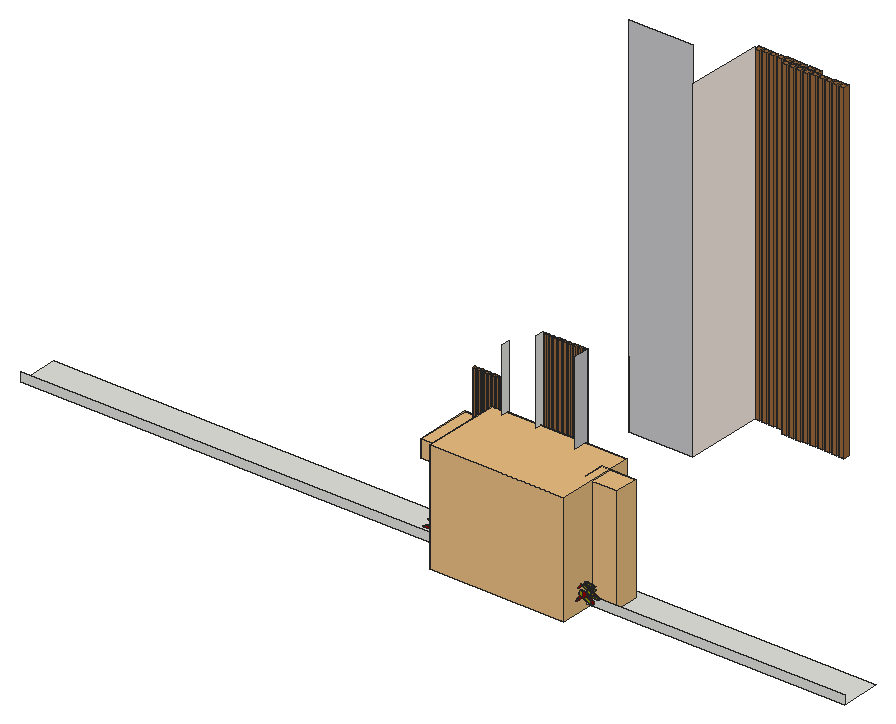
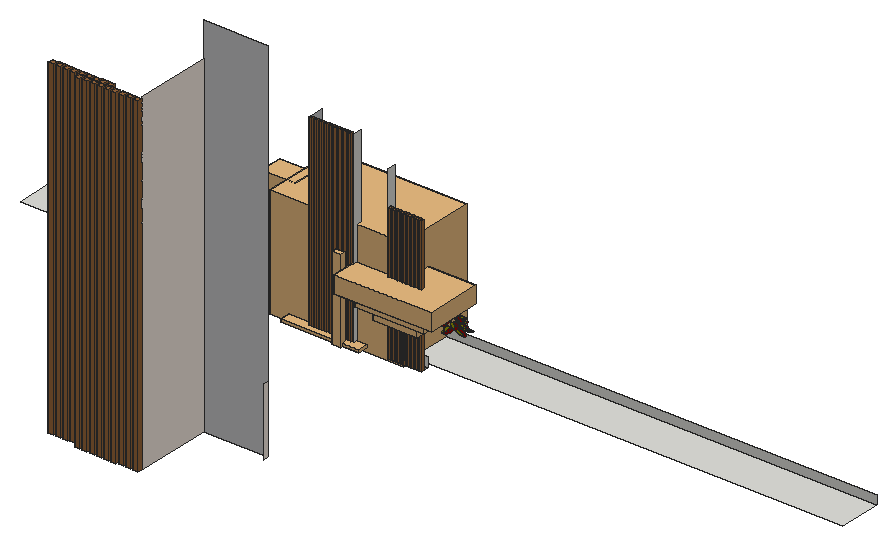
# SketchUp Ruby script. Lengths in inches.
U = 1.inch
M = Sketchup.active_model
def pt(a) = Geom::Point3d.new(a.map { |v| v * U })
def face(e, loops, mat)
  f = e.add_face(loops[0].map { |a| pt(a) })
  loops[1..].each { |l| e.add_face(l.map { |a| pt(a) }).erase! }
  f.material = f.back_material = mat if mat
  f
end
# faces: each face lists its corners as indices into pts; further lists are holes
def faces(e, pts, list, mat = nil) = list.each { |f| face(e, (f[0].is_a?(Array) ? f : [f]).map { |l| l.map { |i| pts[i] } }, mat) }
# xy, xz, yz: faces in a plane at the given z, y or x. An outline is a flat list of corners, or four numbers for a rectangle; further outlines are holes
def ring(l) = l.size == 4 ? [[l[0], l[1]], [l[2], l[1]], [l[2], l[3]], [l[0], l[3]]] : l.each_slice(2).to_a
def flat(e, list, mat, &to3) = list.each { |f| face(e, (f[0].is_a?(Array) ? f : [f]).map { |l| ring(l).map { |u, v| to3.(u, v) } }, mat) }
def xy(e, z, list, mat = nil) = flat(e, list, mat) { |x, y| [x, y, z] }
def xz(e, y, list, mat = nil) = flat(e, list, mat) { |x, z| [x, y, z] }
def yz(e, x, list, mat = nil) = flat(e, list, mat) { |y, z| [x, y, z] }
def lines(e, pts, list) = list.each { |a, b| e.add_line(pt(pts[a]), pt(pts[b])) }
# prism: a flat outline (further loops are holes) pulled along v
def prism(e, loops, v, mat = nil)
  f = face(e, loops, mat); d = Geom::Vector3d.new(v.map { |x| x * U })
  f.pushpull(f.normal.samedirection?(d) ? d.length : -d.length)
end
def box(e, o, s, mat = nil) = prism(e, [[o, [o[0] + s[0], o[1], o[2]], [o[0] + s[0], o[1] + s[1], o[2]], [o[0], o[1] + s[1], o[2]]]], [0, 0, s[2]], mat)
def at(x, y, z, deg = 0) = Geom::Transformation.translation(pt([x, y, z])) * Geom::Transformation.rotation(ORIGIN, Z_AXIS, deg.degrees)
def axes(o, x, y, z) = Geom::Transformation.new([*x, 0, *y, 0, *z, 0, *pt(o).to_a, 1])
def part(name) = M.definitions.add(name)
# library, detail: a bought-in or finely detailed component or shape, given as its bounding box
def library(name, o, s) = part(name).tap { |d| box(d.entities, o, s) }
def detail(e, o, s) = box(e.add_group.entities, o, s)
def put(e, d, t, mat = nil) = e.add_instance(d, t).tap { |i| i.material = mat if mat }
def group(e, t, mat = nil) = e.add_group.tap { |g| g.transformation = t; g.material = mat if mat }.entities
root = M.entities
M.materials.add("[0009_Linen]").color = [250, 240, 230]
M.materials.add("[0022_Maroon]").color = [128, 0, 0]
M.materials.add("[0043_SaddleBrown]").color = [139, 69, 19]
M.materials.add("[0058_Olive]").color = [128, 128, 0]
M.materials.add("[Blacktop Old 01]").color = [132, 136, 139]
M.materials.add("[Polished Concrete New]").color = [200, 200, 203]
M.materials.add("[Wood Floor]").color = [155, 105, 61]
M.materials.add("[Wood Veneer 02]").color = [190, 128, 91]
c1 = part("Group\#46")
p = [[0.46,5.4,1.48],[0.55,4.86,1.35],[0.68,4.33,1.23],[0.85,3.8,1.12],[1.04,3.28,1.02],[1.28,2.78,0.93],
  [1.54,2.29,0.84],[1.84,1.82,0.77],[2.17,1.36,0.71],[2.52,0.93,0.66],[2.91,0.52,0.62],[2.91,0,0.48],
  [2.47,0.44,0.52],[2.06,0.9,0.56],[1.68,1.39,0.625],[1.34,1.9,0.7],[1.03,2.43,0.79],[0.76,2.98,0.89],
  [0.53,3.55,1],[0.34,4.13,1.12],[0.19,4.72,1.25],[0.09,5.3125,1.39],[0.02,5.91,1.54],[0,6.51,1.69],
  [0.02,6.88,1.8],[0.1,7.24,1.91],[0.22,7.59,2.02],[0.39,7.92,2.14],[0.6,8.22,2.26],[0.85,8.49,2.38],
  [1.14,8.72,2.49],[1.45,8.91,2.6],[1.8,9.0625,2.71],[2.16,9.17,2.8],[2.53,9.22,2.88],[2.91,9.23,2.95],
  [2.91,4.61,1.72],[2.68,3.89,1.48],[2.18,2.26,0.95],[2.59,5.625,1.93],[1.61,4.02,1.32],[2.34,6.73,2.18],
  [1.25,5.66,1.69],[2.4,7.87,2.5],[1.14,7.72,2.22],[2.4375,8.83,2.76],[2.16,8.77,2.69],[1.89,8.68,2.62],
  [1.625,8.56,2.54],[1.39,8.42,2.46],[1.16,8.24,2.37],[0.97,8.04,2.28],[0.79,7.82,2.19],[0.65,7.58,2.1],
  [0.54,7.32,2.01],[0.45,7.05,1.92],[0.4,6.78,1.84],[0.39,6.49,1.76],[0.41,5.95,1.62],[5.79,6.88,1.8],
  [5.82,6.51,1.69],[5.79,5.91,1.54],[5.73,5.3125,1.39],[5.625,4.72,1.25],[5.48,4.13,1.12],[5.29,3.55,1],
  [5.06,2.98,0.89],[4.79,2.43,0.79],[4.48,1.9,0.7],[4.14,1.39,0.625],[3.76,0.9,0.56],[3.35,0.44,0.52],
  [3.29,0.93,0.66],[3.65,1.36,0.71],[3.98,1.82,0.77],[4.27,2.29,0.84],[4.54,2.78,0.93],[4.77,3.28,1.02],
  [4.97,3.8,1.12],[5.13,4.33,1.23],[5.26,4.86,1.35],[5.35,5.4,1.48],[5.41,5.95,1.62],[5.43,6.49,1.76],
  [5.41,6.78,1.84],[5.36,7.05,1.92],[5.28,7.32,2.01],[5.16,7.58,2.1],[5.02,7.82,2.19],[4.85,8.04,2.28],
  [4.65,8.24,2.37],[4.43,8.42,2.46],[4.1875,8.56,2.54],[3.93,8.68,2.62],[3.66,8.77,2.69],[3.38,8.83,2.76],
  [4.67,7.72,2.22],[3.41,7.87,2.5],[4.5625,5.66,1.69],[3.47,6.73,2.18],[4.21,4.02,1.32],[3.23,5.625,1.93],
  [3.64,2.26,0.95],[3.13,3.89,1.48],[3.29,9.22,2.88],[3.66,9.17,2.8],[4.02,9.0625,2.71],[4.36,8.91,2.6],
  [4.68,8.72,2.49],[4.96,8.49,2.38],[5.21,8.22,2.26],[5.43,7.92,2.14],[5.59,7.59,2.02],[5.72,7.24,1.91],
  [2.91,14.34,0]]
faces(c1.entities,p,[[0,1,2,3,4,5,6,7,8,9,10,11,12,13,14,15,16,17,18,19,20,21,22,23,24,25,26,27,28,29,30,31,32,33,34,35,36,10,37,38,39,40,41,42,43,44,45,46,47,48,49,50,51,52,53,54,55,56,57,58],[59,60,61,62,63,64,65,66,67,68,69,70,71,11,10,72,73,74,75,76,77,78,79,80,81,82,83,84,85,86,87,88,89,90,91,92,93,94,95,96,97,98,99,100,101,102,103,10,36,35,104,105,106,107,108,109,110,111,112,113]],"[0022_Maroon]")
faces(c1.entities,p,[[43,42,41,40,39,38,37,10,9,8,7,6,5,4,3,2,1,0,58,57,56,55,54,53,52,51,50,49,48,47,46,45,44],[99,98,97,96,95,94,93,92,91,90,89,88,87,86,85,84,83,82,81,80,79,78,77,76,75,74,73,72,10,103,102,101,100]],"[0058_Olive]")
lines(c1.entities,p,[[35,114]])
c2 = part("EXOTIC-CROTON")
p = [[0,0,13.11],[0,0,0],[0,0,17.6]]
lines(c2.entities,p,[[0,1],[0,2]])
put(c2.entities,c1,at(-2.91,-14.34,9.43),"[0058_Olive]")
put(c2.entities,c1,at(-13.875,-4.65,9.43,-60),"[0058_Olive]")
put(c2.entities,c1,at(-10.97,9.69,9.43,-120),"[0058_Olive]")
put(c2.entities,c1,at(2.91,14.34,9.43,180),"[0058_Olive]")
put(c2.entities,c1,at(13.875,4.65,9.43,120),"[0058_Olive]")
put(c2.entities,c1,at(10.97,-9.69,9.43,60),"[0058_Olive]")
put(c2.entities,c1,axes([-3.96,11.79,13.11],[-0.73612,-0.425,0],[0.425,-0.73612,0],[0,0,0.85]),"[0058_Olive]")
put(c2.entities,c1,axes([8.24,9.32,13.11],[-0.73612,0.425,0],[-0.425,-0.73612,0],[0,0,0.85]),"[0058_Olive]")
put(c2.entities,c1,axes([3.96,-11.79,13.11],[0.73612,0.425,0],[-0.425,0.73612,0],[0,0,0.85]),"[0058_Olive]")
put(c2.entities,c1,axes([-8.24,-9.32,13.11],[0.73612,-0.425,0],[0.425,0.73612,0],[0,0,0.85]),"[0058_Olive]")
put(c2.entities,c1,axes([12.19,-2.47,13.11],[0,0.85,0],[-0.85,0,0],[0,0,0.85]),"[0058_Olive]")
put(c2.entities,c1,axes([-12.19,2.47,13.11],[0,-0.85,0],[0.85,0,0],[0,0,0.85]),"[0058_Olive]")
put(c2.entities,c1,axes([1.98,9.75,17.6],[-0.68,0,0],[0,-0.68,0],[0,0,0.68]),"[0058_Olive]")
put(c2.entities,c1,axes([7.46,-6.59,17.6],[0.34,0.5889,0],[-0.5889,0.34,0],[0,0,0.68]),"[0058_Olive]")
put(c2.entities,c1,axes([9.4375,3.16,17.6],[-0.34,0.5889,0],[-0.5889,-0.34,0],[0,0,0.68]),"[0058_Olive]")
put(c2.entities,c1,axes([-9.4375,-3.16,17.6],[0.34,-0.5889,0],[0.5889,0.34,0],[0,0,0.68]),"[0058_Olive]")
put(c2.entities,c1,axes([-7.46,6.59,17.6],[-0.34,-0.5889,0],[0.5889,-0.34,0],[0,0,0.68]),"[0058_Olive]")
put(c2.entities,c1,axes([-1.98,-9.75,17.6],[0.68,0,0],[0,0.68,0],[0,0,0.68]),"[0058_Olive]")
c3 = part("Group\#2")
xy(c3.entities,0,[[0,0,1.85,1.85],[2.64,0,4.49,1.85],[5.28,0,7.125,1.85],[7.91,0,9.76,1.85],[10.55,0,12.4,1.85],
  [13.1875,0,15.04,1.85],[15.83,0,17.68,1.85],[18.46,0,20.31,1.85],[21.1,0,22.95,1.85]],"[Wood Floor]")
g1 = group(c3.entities,at(0,0,0))
xy(g1,112.2,[[0,0,1.85,1.85],[2.64,0,4.49,1.85],[5.28,0,7.125,1.85],[7.91,0,9.76,1.85],[10.55,0,12.4,1.85],
  [13.1875,0,15.04,1.85],[15.83,0,17.68,1.85],[18.46,0,20.31,1.85],[21.1,0,22.95,1.85]],"[Wood Floor]")
xz(g1,0,[[0,0,1.85,112.2],[2.64,0,4.49,112.2],[5.28,0,7.125,112.2],[7.91,0,9.76,112.2],[10.55,0,12.4,112.2],
  [13.1875,0,15.04,112.2],[15.83,0,17.68,112.2],[18.46,0,20.31,112.2],[21.1,0,22.95,112.2]],"[Wood Floor]")
xz(g1,1.85,[[0,0,1.85,112.2],[2.64,0,4.49,112.2],[5.28,0,7.125,112.2],[7.91,0,9.76,112.2],[10.55,0,12.4,112.2],
  [13.1875,0,15.04,112.2],[15.83,0,17.68,112.2],[18.46,0,20.31,112.2],[21.1,0,22.95,112.2]],"[Wood Floor]")
yz(g1,0,[[0,0,1.85,112.2]],"[Wood Floor]")
yz(g1,1.85,[[0,0,1.85,112.2]],"[Wood Floor]")
yz(g1,2.64,[[0,0,1.85,112.2]],"[Wood Floor]")
yz(g1,4.49,[[0,0,1.85,112.2]],"[Wood Floor]")
yz(g1,5.28,[[0,0,1.85,112.2]],"[Wood Floor]")
yz(g1,7.125,[[0,0,1.85,112.2]],"[Wood Floor]")
yz(g1,7.91,[[0,0,1.85,112.2]],"[Wood Floor]")
yz(g1,9.76,[[0,0,1.85,112.2]],"[Wood Floor]")
yz(g1,10.55,[[0,0,1.85,112.2]],"[Wood Floor]")
yz(g1,12.4,[[0,0,1.85,112.2]],"[Wood Floor]")
yz(g1,13.1875,[[0,0,1.85,112.2]],"[Wood Floor]")
yz(g1,15.04,[[0,0,1.85,112.2]],"[Wood Floor]")
yz(g1,15.83,[[0,0,1.85,112.2]],"[Wood Floor]")
yz(g1,17.68,[[0,0,1.85,112.2]],"[Wood Floor]")
yz(g1,18.46,[[0,0,1.85,112.2]],"[Wood Floor]")
yz(g1,20.31,[[0,0,1.85,112.2]],"[Wood Floor]")
yz(g1,21.1,[[0,0,1.85,112.2]],"[Wood Floor]")
yz(g1,22.95,[[0,0,1.85,112.2]],"[Wood Floor]")
c4 = part("Group\#44")
p = [[12.14,1.93,0.52],[12.15,1.96,0.53]]
lines(c4.entities,p,[[0,1]])
detail(c4.entities,[0,0,0],[22.29,22.29,3.9])
c5 = part("EXOTIC-BUSHY-02")
prism(c5.entities,[[[-0.2,0.11,-0.03],[-0.16,0.16,-0.03],[-0.11,0.2,-0.03],[-0.06,0.22,-0.03],[0,0.23,-0.03],[0.06,0.22,-0.03],[0.11,0.2,-0.03],[0.16,0.16,-0.03],[0.2,0.11,-0.03],[0.22,0.06,-0.03],[0.23,0,-0.03],[0.22,-0.06,-0.03],[0.2,-0.11,-0.03],[0.16,-0.16,-0.03],[0.11,-0.2,-0.03],[0.06,-0.22,-0.03],[0,-0.23,-0.03],[-0.06,-0.22,-0.03],[-0.11,-0.2,-0.03],[-0.16,-0.16,-0.03],[-0.2,-0.11,-0.03],[-0.22,-0.06,-0.03],[-0.23,0,-0.03],[-0.22,0.06,-0.03]]],[0,0,12.79],"[0043_SaddleBrown]")
put(c5.entities,c4,axes([-11.15,-11.15,16.66],[1,0,0],[0,1,0],[0,0,-1]))
put(c5.entities,c4,axes([-7.91,-7.91,13.14],[0.71,0,0],[0,0.71,0],[0,0,-0.71]))
put(c5.entities,c4,axes([-5.11,-5.11,9.7],[0.4588,0,0],[0,0.4588,0],[0,0,-0.4588]))
c6 = library("EXOTIC-BULLRUSH",[-0.59,-0.59,-0.94],[7.09,7.09,64.29])
c7 = library("EXOTIC-KENTIA\#1",[0.7,-0.7,-0.11],[104.19,106.14,86.09])
c8 = library("EXOTIC-AMAZON-LILY",[-1.1,-0.12,0],[60.56,66.69,1.97])
c9 = library("EXOTICA-CAT-TAIL",[-18.64,-20.64,0],[26.41,31.25,82.25])
xy(root,0,[[321.78,153.99,347.76,160.36],[373.77,153.99,408.3,160.36]],"[Blacktop Old 01]")
xy(root,0.6875,[[3.82,118.08,641.18,118.08,641.18,148.8,408.3,148.8,408.3,150.16,3.82,150.16]])
xz(root,118.08,[[3.82,0.6875,641.18,7.8125]])
xz(root,148.8,[[408.3,0,454.65,0.6875],[408.3,0.6875,454.65,7.8125]],"[Polished Concrete New]")
xz(root,153.99,[[321.78,0,347.76,7.8125],[373.77,0,408.3,7.8125]])
xz(root,153.99,[[347.76,0,373.77,7.8125]],"[Polished Concrete New]")
xz(root,160.36,[[373.77,0,408.3,146.4375]],"[Wood Veneer 02]")
xz(root,300.43,[[328.15,0,378.25,285.125]],"[Polished Concrete New]")
yz(root,328.15,[[300.43,0,304.24,52.25]],"[0009_Linen]")
yz(root,347.76,[[153.99,0,160.36,131.1875]])
yz(root,373.77,[[153.99,0,160.36,146.4375]])
yz(root,378.25,[[300.43,0,359.87,258.1]],"[0009_Linen]")
yz(root,408.3,[[148.8,0,153.99,0,153.99,7.8125,150.16,7.8125,150.16,0.6875,148.8,0.6875],[148.8,0.6875,150.16,7.8125]])
yz(root,408.3,[[153.99,0,153.99,7.8125,148.8,7.8125,148.8,146.4375,160.36,146.4375,160.36,0]],"[Polished Concrete New]")
put(root,c2,axes([328.33,121.21,0.6875],[1,0,0],[0,0.5735,0],[0,0,1]))
put(root,c3,axes([321.78,160.36,0],[1.13172,0,0],[0,-1.32521,0],[0,0,0.93072]))
put(root,c5,axes([336.68,157.41,0.75],[3.38,0,0],[0,1.93843,0],[0,0,3.38]))
put(root,c2,axes([342.22,119.43,-2.38],[0.783,0,0],[0,0.44905,0],[0,0,0.783]))
put(root,c6,axes([379.16,163.41,0.6875],[1,0,0],[0,0.5735,0],[0,0,1]))
put(root,c7,axes([336.11,97.65,-2.89],[1,0,0],[0,0.5735,0],[0,0,1]))
put(root,c3,axes([375.57,159.11,0],[1.42597,0,0],[0,1.00934,0],[0,0,1.30509]))
put(root,c8,axes([366.51,128.21,0.6875],[1,0,0],[0,0.5735,0],[0,0,1]))
put(root,c3,axes([378.25,359.87,0],[2.12,0,0],[0,2.12,0],[0,0,2.2896]))
put(root,c3,axes([402.02,355.95,0],[2.12,0,0],[0,2.12,0],[0,0,2.2896]))
put(root,c2,axes([426.89,112.96,-5.96],[0.783,0,0],[0,0.44905,0],[0,0,0.783]))
put(root,c2,axes([440.51,114.75,-2.89],[1,0,0],[0,0.5735,0],[0,0,1]))
put(root,c9,axes([452.85,135.64,0.6875],[1,0,0],[0,0.5735,0],[0,0,1]))
